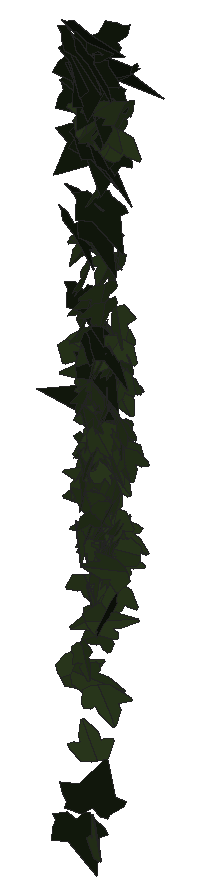
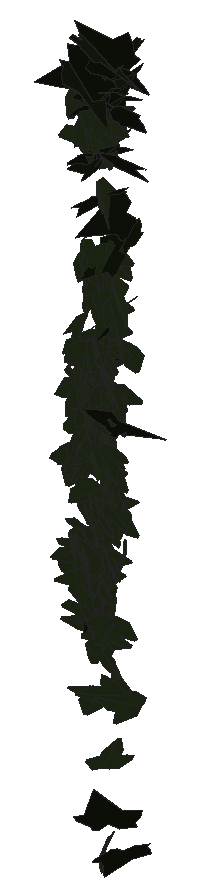
# SketchUp Ruby script. Lengths in inches.
U = 1.inch
M = Sketchup.active_model
def pt(a) = Geom::Point3d.new(a.map { |v| v * U })
def face(e, loops, mat)
  f = e.add_face(loops[0].map { |a| pt(a) })
  loops[1..].each { |l| e.add_face(l.map { |a| pt(a) }).erase! }
  f.material = f.back_material = mat if mat
  f
end
# faces: each face lists its corners as indices into pts; further lists are holes
def faces(e, pts, list, mat = nil) = list.each { |f| face(e, (f[0].is_a?(Array) ? f : [f]).map { |l| l.map { |i| pts[i] } }, mat) }
# xy, xz, yz: faces in a plane at the given z, y or x. An outline is a flat list of corners, or four numbers for a rectangle; further outlines are holes
def ring(l) = l.size == 4 ? [[l[0], l[1]], [l[2], l[1]], [l[2], l[3]], [l[0], l[3]]] : l.each_slice(2).to_a
def flat(e, list, mat, &to3) = list.each { |f| face(e, (f[0].is_a?(Array) ? f : [f]).map { |l| ring(l).map { |u, v| to3.(u, v) } }, mat) }
def xy(e, z, list, mat = nil) = flat(e, list, mat) { |x, y| [x, y, z] }
def xz(e, y, list, mat = nil) = flat(e, list, mat) { |x, z| [x, y, z] }
def yz(e, x, list, mat = nil) = flat(e, list, mat) { |y, z| [x, y, z] }
def lines(e, pts, list) = list.each { |a, b| e.add_line(pt(pts[a]), pt(pts[b])) }
# prism: a flat outline (further loops are holes) pulled along v
def prism(e, loops, v, mat = nil)
  f = face(e, loops, mat); d = Geom::Vector3d.new(v.map { |x| x * U })
  f.pushpull(f.normal.samedirection?(d) ? d.length : -d.length)
end
def box(e, o, s, mat = nil) = prism(e, [[o, [o[0] + s[0], o[1], o[2]], [o[0] + s[0], o[1] + s[1], o[2]], [o[0], o[1] + s[1], o[2]]]], [0, 0, s[2]], mat)
def at(x, y, z, deg = 0) = Geom::Transformation.translation(pt([x, y, z])) * Geom::Transformation.rotation(ORIGIN, Z_AXIS, deg.degrees)
def axes(o, x, y, z) = Geom::Transformation.new([*x, 0, *y, 0, *z, 0, *pt(o).to_a, 1])
def part(name) = M.definitions.add(name)
# library, detail: a bought-in or finely detailed component or shape, given as its bounding box
def library(name, o, s) = part(name).tap { |d| box(d.entities, o, s) }
def detail(e, o, s) = box(e.add_group.entities, o, s)
def put(e, d, t, mat = nil) = e.add_instance(d, t).tap { |i| i.material = mat if mat }
def group(e, t, mat = nil) = e.add_group.tap { |g| g.transformation = t; g.material = mat if mat }.entities
root = M.entities
M.materials.add("1026 AP 7946 SUNNY SIDE UP").color = [254, 231, 186]
M.materials.add("efeu1").color = [18, 25, 13]
M.materials.add("efeu2").color = [43, 57, 29]
c1 = part("ivyleaf_10")
p = [[0,0.5,-0.03],[-0.0625,2.02,-0.43],[-0.19,2.01,-0.46],[-0.54,1.05,-0.29],[-0.52,0.625,-0.18],[-0.83,0.76,-0.28],
  [-1.16,0.64,-0.33],[-1.15,0.33,-0.24],[-0.77,-0.39,0.02],[-0.3,-0.51,0.16],[0.04,-0.48,0.23],[-0.02,2.01,-0.4375],
  [-0.06,2.01,-0.43],[0.04,-0.49,0.23],[0.67,-0.49,0.14],[1.38,0.36,-0.2],[1.375,0.51,-0.24],[0.81,0.65,-0.19],
  [0.62,0.59,-0.15],[0.6,1.09,-0.28],[0.5,1.23,-0.31]]
faces(c1.entities,p,[[0,1,2,3,4,5,6,7,8,9,10],[11,12,0,13,14,15,16,17,18,19,20]],"efeu2")
c2 = part("ivyleaf_9")
p = [[1.54,2.16,1.25],[1.36,2.04,1.19],[-0.21,0.99,0.68],[-0.71,1.11,0.82],[-0.85,0.86,0.67],[-0.8,0.17,0.21],
  [-0.9,-0.01,0.1],[-0.67,-0.16,-0.02],[-0.08,-0.08,-0.05],[-0.03,-0.6,-0.4],[0.65,-0.88,-0.66],[0.83,-0.6,-0.49],
  [1.29,-0.42,-0.43],[1.8125,-0.07,-0.26],[1.21,0.44,0.15]]
faces(c2.entities,p,[[0,1,2,3,4,5,6,7,8,9,10,11,12,13,14]],"efeu1")
put(root,c1,axes([106.875,212.88,260.41],[-0.19029,-0.14773,0.11261],[-0.06597,-0.10624,-0.19489],[0.28215,-0.12447,0.03039]),"1026 AP 7946 SUNNY SIDE UP")
put(root,c2,axes([107.1,212.89,261.68],[-0.24512,0.04227,0.19567],[-0.3019,0.00418,-0.16348],[-0.04735,-0.24549,0.02942]),"1026 AP 7946 SUNNY SIDE UP")
put(root,c1,axes([106.83,212.86,260.92],[-0.31168,0.09367,0.01752],[-0.03684,-0.01117,-0.22498],[-0.14494,-0.19859,0.0195]),"1026 AP 7946 SUNNY SIDE UP")
put(root,c1,axes([106.73,212.96,258.57],[-0.26839,-0.09301,-0.07264],[0.13434,-0.01575,-0.19319],[0.12429,-0.1838,0.05196]),"1026 AP 7946 SUNNY SIDE UP")
put(root,c1,axes([106.63,212.64,257.13],[0.09438,0.04793,-0.22139],[0.24114,0.15113,0.07963],[0.24902,-0.16451,0.0068]),"1026 AP 7946 SUNNY SIDE UP")
put(root,c1,axes([106.8125,212.81,260.76],[0.22467,-0.16796,0.00881],[-0.00657,-0.01601,-0.22684],[0.26444,0.1423,-0.01312]),"1026 AP 7946 SUNNY SIDE UP")
put(root,c1,axes([106.83,212.74,263.82],[0.11401,-0.23435,0.00026],[0.0017,-0.00132,-0.25272],[0.3685,0.07251,0.00109]),"1026 AP 7946 SUNNY SIDE UP")
put(root,c2,axes([106.7,212.92,267.24],[-0.06033,-0.19698,0.16164],[0.02129,-0.16121,-0.20458],[0.39651,-0.02131,0.03558]),"1026 AP 7946 SUNNY SIDE UP")
put(root,c1,axes([106.82,212.73,260.82],[-0.08581,0.21184,0.03996],[-0.04434,0.0314,-0.22431],[-0.33538,-0.05835,0.01943]),"1026 AP 7946 SUNNY SIDE UP")
put(root,c1,axes([106.86,212.83,262.19],[-0.24604,-0.16556,0.00822],[0.00748,-0.01674,-0.23427],[0.26059,-0.15583,0.01449]),"1026 AP 7946 SUNNY SIDE UP")
put(root,c1,axes([106.86,212.9,260.92],[-0.00747,-0.22363,-0.00585],[-0.00483,0.00447,-0.23038],[0.35166,-0.00469,-0.00329]),"1026 AP 7946 SUNNY SIDE UP")
put(root,c1,axes([106.77,212.95,262.59],[-0.16197,0.17997,-0.09615],[0.04265,-0.09266,-0.21312],[-0.31666,-0.10453,0.02047]),"1026 AP 7946 SUNNY SIDE UP")
put(root,c2,axes([106.64,212.77,267.67],[0.15307,-0.24266,0.02043],[-0.00058,-0.02299,-0.26933],[0.38301,0.09694,-0.00857]),"1026 AP 7946 SUNNY SIDE UP")
put(root,c2,axes([106.95,212.89,266.02],[-0.3785,-0.06932,-0.00194],[0.02255,-0.04449,-0.25379],[0.10667,-0.23657,0.04675]),"1026 AP 7946 SUNNY SIDE UP")
put(root,c1,axes([106.82,212.9,258.9],[-0.21299,0.15516,-0.01584],[0.00136,-0.02078,-0.21188],[-0.2453,-0.13483,0.01258]),"1026 AP 7946 SUNNY SIDE UP")
put(root,c1,axes([106.76,212.7,259.54],[-0.0639,0.19851,-0.12817],[0.03544,-0.12353,-0.20945],[-0.36761,-0.04642,0.00209]),"1026 AP 7946 SUNNY SIDE UP")
put(root,c1,axes([106.83,212.96,259.66],[0.14342,-0.19112,0.02627],[0.01622,-0.02453,-0.2183],[0.30298,0.09178,-0.00075]),"1026 AP 7946 SUNNY SIDE UP")
put(root,c1,axes([106.87,212.97,259.56],[-0.16054,-0.18227,0.03579],[0.01037,-0.04436,-0.21367],[0.29189,-0.09868,0.02728]),"1026 AP 7946 SUNNY SIDE UP")
put(root,c1,axes([106.89,212.85,264.41],[-0.02994,-0.19682,0.14607],[-0.01596,-0.14258,-0.20452],[0.38213,-0.02137,0.0029]),"1026 AP 7946 SUNNY SIDE UP")
put(root,c1,axes([106.89,213,259.29],[-0.09176,-0.19462,0.03705],[-0.00634,-0.03747,-0.20942],[0.31146,-0.0581,0.00666]),"1026 AP 7946 SUNNY SIDE UP")
put(root,c1,axes([106.86,212.93,264.49],[-0.1538,-0.22251,-0.06366],[0.05442,0.05085,-0.24985],[0.35848,-0.10318,0.01061]),"1026 AP 7946 SUNNY SIDE UP")
put(root,c1,axes([106.82,212.9,258.44],[-0.09357,0.19403,-0.03018],[0.00656,-0.03051,-0.20919],[-0.30874,-0.05945,0.0047]),"1026 AP 7946 SUNNY SIDE UP")
put(root,c2,axes([106.66,212.73,264.58],[0.10039,-0.19777,0.14375],[0.06086,-0.13528,-0.21485],[0.37671,0.07456,-0.0036]),"1026 AP 7946 SUNNY SIDE UP")
put(root,c2,axes([106.79,212.83,266.9],[-0.05764,-0.12549,0.22384],[-0.03673,-0.21764,-0.1344],[0.3938,-0.03867,0.02023]),"1026 AP 7946 SUNNY SIDE UP")
put(root,c2,axes([106.7,212.9,264.57],[0.32306,-0.13253,-0.05726],[-0.07283,0.02935,-0.2517],[0.21344,0.21061,0.00078]),"1026 AP 7946 SUNNY SIDE UP")
put(root,c1,axes([106.9,212.66,263.17],[0.12332,-0.21752,-0.044],[0.0002,0.04404,-0.23746],[0.34819,0.07701,0.01572]),"1026 AP 7946 SUNNY SIDE UP")
put(root,c1,axes([106.88,212.91,260.07],[-0.29785,0.09958,-0.02522],[0.02592,-0.02239,-0.22025],[-0.15936,-0.18976,0.01132]),"1026 AP 7946 SUNNY SIDE UP")
put(root,c1,axes([107.06,212.62,262.05],[-0.27734,0.09266,0.12943],[-0.20342,0.01796,-0.20148],[-0.1362,-0.2155,0.03736]),"1026 AP 7946 SUNNY SIDE UP")
put(root,c1,axes([106.89,212.76,260.12],[-0.32683,-0.04574,-0.03259],[0.05394,-0.01036,-0.21859],[0.06855,-0.20995,0.0166]),"1026 AP 7946 SUNNY SIDE UP")
put(root,c2,axes([106.7,212.76,265.12],[0.36817,-0.07574,-0.00511],[-0.00424,0.00639,-0.25343],[0.11924,0.2341,0.00678]),"1026 AP 7946 SUNNY SIDE UP")
put(root,c2,axes([106.79,212.64,254.71],[-0.0297,-0.22602,-0.09822],[0.02553,0.09298,-0.23297],[0.38409,-0.02365,0.00789]),"1026 AP 7946 SUNNY SIDE UP")
put(root,c1,axes([106.89,212.97,259.24],[-0.07735,-0.19475,0.04909],[0.08021,-0.06068,-0.19702],[0.30533,-0.0334,0.0642]),"1026 AP 7946 SUNNY SIDE UP")
put(root,c1,axes([106.96,212.67,261.98],[0.03385,-0.23664,0.016],[-0.00236,-0.01708,-0.24488],[0.37304,0.02137,-0.003]),"1026 AP 7946 SUNNY SIDE UP")
put(root,c1,axes([106.93,212.8,262.29],[0.17732,-0.20113,0.02047],[0.00895,-0.02089,-0.23761],[0.31785,0.11279,-0.00473]),"1026 AP 7946 SUNNY SIDE UP")
put(root,c1,axes([106.95,212.56,260.36],[0.14897,-0.18169,-0.09819],[-0.01013,0.10119,-0.20697],[0.3217,0.08732,0.03895]),"1026 AP 7946 SUNNY SIDE UP")
put(root,c1,axes([106.92,212.92,262.8],[-0.04274,0.22618,0.01962],[-0.03349,0.01526,-0.23376],[-0.35517,-0.02866,0.01968]),"1026 AP 7946 SUNNY SIDE UP")
put(root,c1,axes([106.97,212.94,261.29],[0.33624,0.00031,-0.06747],[-0.10153,0.03846,-0.21677],[0.01725,0.22031,0.03926]),"1026 AP 7946 SUNNY SIDE UP")
put(root,c1,axes([106.98,212.65,263.45],[-0.02373,-0.23584,-0.00858],[0.00184,0.00693,-0.24341],[0.37099,-0.01512,0.00066]),"1026 AP 7946 SUNNY SIDE UP")
put(root,c1,axes([107.05,212.86,258.17],[0.0938,0.07416,-0.18861],[-0.19686,-0.1343,-0.09863],[-0.24103,0.13855,0.00716]),"1026 AP 7946 SUNNY SIDE UP")
put(root,c1,axes([106.97,212.71,260.84],[0.04979,-0.16342,-0.17953],[0.01601,0.17564,-0.16764],[0.37425,0.01423,0.03106]),"1026 AP 7946 SUNNY SIDE UP")
put(root,c1,axes([106.78,212.72,257.55],[0.19392,-0.06096,0.15494],[0.20835,-0.07198,-0.14209],[0.1482,0.18098,-0.00298]),"1026 AP 7946 SUNNY SIDE UP")
put(root,c1,axes([106.97,212.81,266.59],[-0.13246,-0.18428,0.15838],[0.04374,-0.17036,-0.19433],[0.37588,-0.04511,0.07843]),"1026 AP 7946 SUNNY SIDE UP")
put(root,c1,axes([106.92,213,259.3],[-0.08049,0.14506,-0.14378],[0.01611,-0.14278,-0.15667],[-0.31701,-0.04409,0.02855]),"1026 AP 7946 SUNNY SIDE UP")
put(root,c1,axes([107.08,212.98,259.58],[-0.30723,0.00362,0.07405],[-0.11153,-0.04462,-0.19662],[0.019,-0.20335,0.04321]),"1026 AP 7946 SUNNY SIDE UP")
put(root,c2,axes([107.24,212.93,267.75],[-0.28959,0.17928,0.02162],[-0.0941,-0.0338,-0.25617],[-0.26758,-0.18214,0.06669]),"1026 AP 7946 SUNNY SIDE UP")
put(root,c1,axes([106.91,213.01,259.29],[0.20346,-0.14102,0.08381],[0.08078,-0.06432,-0.19747],[0.24358,0.13912,-0.00452]),"1026 AP 7946 SUNNY SIDE UP")
put(root,c1,axes([107.17,212.75,257.9375],[-0.20498,0.0587,0.15321],[-0.24335,0.00021,-0.14015],[-0.06117,-0.19752,0.04412]),"1026 AP 7946 SUNNY SIDE UP")
put(root,c1,axes([106.99,212.89,262.75],[0.162,-0.205,0.01846],[-0.00097,-0.02164,-0.23625],[0.32374,0.10252,-0.00994]),"1026 AP 7946 SUNNY SIDE UP")
put(root,c2,axes([106.83,212.74,263.5],[0.07723,-0.23826,-0.01681],[0.00159,0.01549,-0.25049],[0.37537,0.04895,0.00452]),"1026 AP 7946 SUNNY SIDE UP")
put(root,c2,axes([106.71,212.93,267.61],[0.03453,-0.11597,0.23289],[0.26498,-0.16399,-0.10419],[0.30021,0.15809,0.06517]),"1026 AP 7946 SUNNY SIDE UP")
put(root,c1,axes([107.01,212.9375,259.71],[0.11923,-0.2002,-0.02236],[-0.00484,0.02082,-0.22037],[0.31641,0.07576,0.00505]),"1026 AP 7946 SUNNY SIDE UP")
put(root,c2,axes([106.88,212.81,266.79],[-0.23049,-0.12029,-0.17045],[0.22534,0.08369,-0.19379],[0.22831,-0.20404,0.01919]),"1026 AP 7946 SUNNY SIDE UP")
put(root,c1,axes([107.02,212.5625,261.65],[-0.28885,0.13019,0.00558],[-0.02396,-0.01345,-0.23114],[-0.20344,-0.18327,0.0193]),"1026 AP 7946 SUNNY SIDE UP")
put(root,c1,axes([106.97,213.02,259.32],[-0.10353,0.19599,-0.02435],[0.00237,-0.02559,-0.21303],[-0.31061,-0.06552,0.00649]),"1026 AP 7946 SUNNY SIDE UP")
put(root,c1,axes([107.22,212.73,262.71],[0.03844,-0.00163,-0.25329],[-0.24968,0.18853,-0.01645],[0.29516,0.15969,0.01907]),"1026 AP 7946 SUNNY SIDE UP")
put(root,c1,axes([107.24,212.9,260.26],[0.10419,-0.06817,-0.23777],[-0.27386,0.15104,-0.09675],[0.2603,0.18619,-0.00662]),"1026 AP 7946 SUNNY SIDE UP")
put(root,c1,axes([107.05,212.88,262.89],[0.06171,-0.23228,-0.00252],[0.0013,0.00128,-0.24268],[0.36524,0.03924,0.00129]),"1026 AP 7946 SUNNY SIDE UP")
put(root,c1,axes([106.84,212.53,262.75],[-0.16671,-0.10976,-0.18567],[0.29094,0.04728,-0.14201],[0.15779,-0.20314,0.06567]),"1026 AP 7946 SUNNY SIDE UP")
put(root,c2,axes([106.87,212.72,266.16],[0.19454,-0.21273,-0.07781],[-0.05362,0.06614,-0.25311],[0.35025,0.12828,0.00447]),"1026 AP 7946 SUNNY SIDE UP")
put(root,c1,axes([107.06,212.9,261.09],[0.06259,-0.21767,0.03943],[0.01034,-0.03896,-0.22818],[0.3477,0.04034,-0.00031]),"1026 AP 7946 SUNNY SIDE UP")
put(root,c1,axes([107.09,212.88,261.91],[-0.17518,-0.18259,0.08696],[0.00076,-0.09787,-0.21537],[0.31698,-0.10067,0.04858]),"1026 AP 7946 SUNNY SIDE UP")
put(root,c2,axes([107.07,212.9,266.96],[-0.29119,-0.17519,0.01232],[0.0312,-0.03955,-0.25921],[0.27445,-0.18138,0.04253]),"1026 AP 7946 SUNNY SIDE UP")
put(root,c2,axes([106.98,212.69,267.38],[-0.30916,-0.08232,-0.16531],[0.24271,0.04461,-0.2188],[0.14539,-0.24953,0.01375]),"1026 AP 7946 SUNNY SIDE UP")
put(root,c1,axes([107.1,212.79,266.3],[-0.01825,-0.25506,0.02821],[-0.00073,-0.02884,-0.2632],[0.40361,-0.01158,0.0008]),"1026 AP 7946 SUNNY SIDE UP")
put(root,c1,axes([107.08,212.77,265.34],[0.0921,-0.24595,-0.02436],[-0.00258,0.02248,-0.2603],[0.3883,0.05848,0.00405]),"1026 AP 7946 SUNNY SIDE UP")
put(root,c1,axes([107.11,212.59,263.06],[-0.0779,-0.23396,-0.03149],[0.00821,0.02878,-0.2462],[0.37066,-0.04981,-0.00116]),"1026 AP 7946 SUNNY SIDE UP")
put(root,c1,axes([107.07,212.7,262.81],[-0.17999,0.20583,-0.00602],[-0.01103,-0.01192,-0.24239],[-0.32365,-0.11406,0.01161]),"1026 AP 7946 SUNNY SIDE UP")
put(root,c1,axes([107.18,212.84,262.82],[0.13309,-0.16861,-0.1382],[-0.11654,0.11145,-0.19322],[0.31712,0.11172,-0.01301]),"1026 AP 7946 SUNNY SIDE UP")
put(root,c1,axes([107.12,212.6,256.01],[0.15553,0.208,0.0165],[-0.02774,-0.00801,0.23688],[0.32671,-0.0997,0.01226]),"1026 AP 7946 SUNNY SIDE UP")
put(root,c2,axes([107.07,212.64,255.08],[-0.27132,-0.05023,0.17508],[0.25865,0.04391,0.18538],[-0.10482,0.23838,0.00425]),"1026 AP 7946 SUNNY SIDE UP")
put(root,c1,axes([107.16,212.73,262.78],[-0.2758,-0.14165,0.03983],[-0.02967,-0.03925,-0.23171],[0.2293,-0.17545,0.01793]),"1026 AP 7946 SUNNY SIDE UP")
put(root,c1,axes([107.14,212.98,258.99],[-0.06114,-0.20357,0.01763],[0.00268,-0.01892,-0.21355],[0.32137,-0.03857,0.00514]),"1026 AP 7946 SUNNY SIDE UP")
put(root,c1,axes([107.08,212.86,259.31],[0.20451,-0.15025,0.05997],[0.03929,-0.0562,-0.20428],[0.25079,0.13132,-0.01689]),"1026 AP 7946 SUNNY SIDE UP")
put(root,c1,axes([107.15,212.93,261.85],[-0.13403,-0.21096,-0.0025],[0.01138,-0.0016,-0.23429],[0.33152,-0.08524,0.00703]),"1026 AP 7946 SUNNY SIDE UP")
put(root,c2,axes([106.9,212.77,267.48],[0.10752,-0.21467,0.13759],[0.07275,-0.12668,-0.23279],[0.39186,0.08242,0.00546]),"1026 AP 7946 SUNNY SIDE UP")
put(root,c1,axes([107.12,212.78,258.91],[0.0614,0.18786,-0.08039],[-0.048,-0.07425,-0.1976],[-0.3169,0.04764,0.01435]),"1026 AP 7946 SUNNY SIDE UP")
put(root,c1,axes([106.89,212.64,257.18],[0.05133,0.02548,0.22125],[0.2849,0.1151,-0.0418],[-0.18526,0.18407,-0.00297]),"1026 AP 7946 SUNNY SIDE UP")
put(root,c1,axes([107.11,212.69,261.49],[0.08141,-0.18179,0.13574],[0.0745,-0.12441,-0.19521],[0.34606,0.06955,0.01009]),"1026 AP 7946 SUNNY SIDE UP")
put(root,c1,axes([107.19,213.01,259.56],[-0.07523,-0.20378,0.0043],[-0.00052,-0.0054,-0.21567],[0.32053,-0.04783,0.00066]),"1026 AP 7946 SUNNY SIDE UP")
put(root,c1,axes([107.22,212.8,266.6875],[-0.07824,-0.22061,0.11325],[-0.03212,-0.10935,-0.23359],[0.38713,-0.05366,0.00351]),"1026 AP 7946 SUNNY SIDE UP")
put(root,c1,axes([107.2,212.76,262.13],[-0.11758,-0.21683,0.03231],[-0.00682,-0.03297,-0.23639],[0.34471,-0.07462,0.00635]),"1026 AP 7946 SUNNY SIDE UP")
put(root,c1,axes([107.19,212.6875,266.42],[0.37106,-0.03707,-0.08098],[-0.10906,0.05575,-0.24191],[0.08186,0.24234,0.04479]),"1026 AP 7946 SUNNY SIDE UP")
put(root,c1,axes([107.1875,212.98,262.85],[-0.25351,-0.16099,0.02945],[0.02995,-0.05958,-0.22808],[0.2556,-0.15269,0.05593]),"1026 AP 7946 SUNNY SIDE UP")
put(root,c1,axes([107.18,213.01,259.55],[0.07349,-0.20198,-0.03268],[-0.0014,0.03117,-0.2133],[0.32121,0.04634,0.00655]),"1026 AP 7946 SUNNY SIDE UP")
put(root,c2,axes([107.34,212.86,267.18],[-0.05532,0.25314,0.0332],[-0.07577,0.02392,-0.2592],[-0.39375,-0.04017,0.04521]),"1026 AP 7946 SUNNY SIDE UP")
put(root,c1,axes([107.18,212.9,260.43],[0.21458,-0.16901,-0.02442],[-0.02544,0.01617,-0.22368],[0.26693,0.1374,-0.00169]),"1026 AP 7946 SUNNY SIDE UP")
put(root,c2,axes([107.1,212.89,266.01],[-0.13414,-0.23643,-0.00553],[0.01675,0.00043,-0.25874],[0.37144,-0.08541,0.00967]),"1026 AP 7946 SUNNY SIDE UP")
put(root,c1,axes([107.15,212.7,262.6875],[0.14328,-0.19688,0.09873],[0.0589,-0.08948,-0.22399],[0.34001,0.09847,-0.0028]),"1026 AP 7946 SUNNY SIDE UP")
put(root,c2,axes([107.09,212.93,266.84],[-0.08432,-0.2459,0.02286],[0.00011,-0.02415,-0.25936],[0.38843,-0.05337,0.00504]),"1026 AP 7946 SUNNY SIDE UP")
put(root,c1,axes([107.22,213.01,259.59],[-0.02747,-0.20842,0.01169],[-0.00606,-0.01225,-0.21552],[0.32825,-0.01767,-0.003]),"1026 AP 7946 SUNNY SIDE UP")
put(root,c2,axes([107.12,212.59,262.97],[0.13523,-0.14255,-0.18512],[-0.15561,0.14911,-0.17056],[0.32426,0.13101,-0.00465]),"1026 AP 7946 SUNNY SIDE UP")
put(root,c1,axes([106.96,212.75,261.02],[-0.09203,-0.06623,-0.2144],[0.31776,0.0643,-0.0794],[0.12876,-0.20603,0.0427]),"1026 AP 7946 SUNNY SIDE UP")
put(root,c1,axes([107.22,213,259.28],[-0.02563,-0.20565,0.0269],[0.00041,-0.02738,-0.21267],[0.3262,-0.01612,0.00238]),"1026 AP 7946 SUNNY SIDE UP")
put(root,c1,axes([107.21,212.88,261.83],[0.03809,-0.2255,0.0098],[0.00767,-0.01033,-0.23368],[0.3549,0.02443,0.004]),"1026 AP 7946 SUNNY SIDE UP")
put(root,c1,axes([107.2,212.8,259.02],[0.22232,-0.16087,-0.01417],[-0.02177,0.00492,-0.22049],[0.25282,0.14189,-0.00652]),"1026 AP 7946 SUNNY SIDE UP")
put(root,c1,axes([107.27,212.49,254.45],[-0.08543,0.1937,-0.1355],[-0.0465,0.1294,0.20794],[0.3662,0.06162,-0.00521]),"1026 AP 7946 SUNNY SIDE UP")
put(root,c2,axes([107.0625,212.71,262.51],[0.05585,-0.22889,-0.08197],[-0.00993,0.0782,-0.2381],[0.38024,0.03566,0.00582]),"1026 AP 7946 SUNNY SIDE UP")
put(root,c1,axes([107.23,212.84,260.05],[0.13016,-0.20435,0.00486],[-0.00752,-0.00827,-0.22705],[0.32137,0.08257,-0.00728]),"1026 AP 7946 SUNNY SIDE UP")
put(root,c1,axes([107.16,212.55,262.8],[-0.12917,-0.17984,-0.1477],[0.14105,0.11396,-0.201],[0.33192,-0.11842,0.02794]),"1026 AP 7946 SUNNY SIDE UP")
put(root,c1,axes([107.28,212.85,262.07],[-0.20871,-0.1812,0.0343],[-0.01494,-0.03551,-0.23121],[0.28961,-0.13242,0.01279]),"1026 AP 7946 SUNNY SIDE UP")
put(root,c1,axes([107.1875,212.5,260.07],[-0.11439,-0.15666,-0.15218],[0.10712,0.13018,-0.1771],[0.32017,-0.09953,0.00488]),"1026 AP 7946 SUNNY SIDE UP")
put(root,c1,axes([107.3,212.9375,262.18],[-0.35423,-0.02409,0.03508],[-0.04876,-0.02951,-0.23207],[0.04414,-0.22594,0.0252]),"1026 AP 7946 SUNNY SIDE UP")
put(root,c1,axes([107.27,212.6,262.63],[0.1028,-0.22374,-0.05806],[-0.01542,0.05451,-0.23974],[0.36199,0.06586,0.00628]),"1026 AP 7946 SUNNY SIDE UP")
put(root,c1,axes([107.29,212.83,264.2],[-0.0978,-0.21205,0.09785],[-0.00278,-0.09913,-0.22688],[0.36611,-0.05739,0.02441]),"1026 AP 7946 SUNNY SIDE UP")
put(root,c1,axes([107.29,212.61,263.8],[-0.10182,-0.22992,-0.01563],[0.00735,0.01309,-0.246],[0.36211,-0.06491,0.0006]),"1026 AP 7946 SUNNY SIDE UP")
put(root,c2,axes([107.1,212.65,264.79],[0.08713,-0.23705,-0.01763],[-0.00003,0.01619,-0.25067],[0.37356,0.05529,0.00409]),"1026 AP 7946 SUNNY SIDE UP")
put(root,c1,axes([107.05,212.94,260.625],[0.2289,0.09188,0.14302],[0.19724,0.05967,-0.1765],[-0.17107,0.19173,-0.01212]),"1026 AP 7946 SUNNY SIDE UP")
put(root,c1,axes([107.28,212.89,266.38],[-0.06047,-0.2493,0.00616],[0.02703,-0.01011,-0.25922],[0.39124,-0.03783,0.01886]),"1026 AP 7946 SUNNY SIDE UP")
put(root,c1,axes([107.49,212.99,259.29],[-0.00746,0.03085,0.21272],[-0.28659,-0.10098,0.01065],[0.15954,-0.17996,0.02908]),"1026 AP 7946 SUNNY SIDE UP")
put(root,c1,axes([107.31,212.59,263.52],[-0.09815,-0.22993,-0.01984],[0.0102,0.01684,-0.24534],[0.3625,-0.06273,0.00153]),"1026 AP 7946 SUNNY SIDE UP")
put(root,c1,axes([107.23,212.5625,261.39],[0.06965,0.2026,0.09348],[-0.01668,0.0932,-0.21118],[-0.34792,0.03609,0.02884]),"1026 AP 7946 SUNNY SIDE UP")
put(root,c1,axes([107.43,212.8125,261.48],[-0.21307,0.13563,0.12354],[-0.20559,0.029,-0.18702],[-0.19574,-0.17809,0.06196]),"1026 AP 7946 SUNNY SIDE UP")
put(root,c1,axes([107.33,212.87,261.5],[-0.32432,0.08555,0.02621],[-0.04454,-0.00329,-0.22961],[-0.13285,-0.20773,0.013]),"1026 AP 7946 SUNNY SIDE UP")
put(root,c1,axes([107.31,212.875,262.53],[0.09771,-0.21477,-0.0741],[-0.00181,0.07302,-0.22913],[0.35553,0.0594,0.0192]),"1026 AP 7946 SUNNY SIDE UP")
put(root,c1,axes([107.31,212.84,266.22],[0.38207,0.03259,-0.06362],[-0.09747,-0.00368,-0.25254],[-0.05109,0.25072,0.00606]),"1026 AP 7946 SUNNY SIDE UP")
put(root,c2,axes([107.08,212.81,265.91],[0.20505,-0.21771,0.02302],[0.00589,-0.02522,-0.2614],[0.34428,0.1301,-0.00924]),"1026 AP 7946 SUNNY SIDE UP")
put(root,c1,axes([107.27,212.95,258.6],[0.32488,-0.00667,-0.01952],[-0.03048,-0.01605,-0.21237],[0.00812,0.20685,-0.01589]),"1026 AP 7946 SUNNY SIDE UP")
put(root,c1,axes([107.375,212.92,262.64],[-0.25913,0.14539,0.07086],[-0.11111,0.02172,-0.22427],[-0.22657,-0.17693,0.02894]),"1026 AP 7946 SUNNY SIDE UP")
put(root,c1,axes([107.33,212.9,262.48],[-0.00387,-0.22559,-0.04368],[0.01512,0.04099,-0.23199],[0.36025,-0.00415,0.00927]),"1026 AP 7946 SUNNY SIDE UP")
put(root,c1,axes([107.26,212.97,259.12],[0.23499,0.14417,0.01405],[-0.00011,0.01851,-0.21337],[-0.22759,0.14885,0.01462]),"1026 AP 7946 SUNNY SIDE UP")
put(root,c2,axes([107.16,212.66,265.19],[0.02014,-0.23537,-0.08176],[0.03964,0.07896,-0.24066],[0.38788,0.00415,0.02884]),"1026 AP 7946 SUNNY SIDE UP")
put(root,c2,axes([107.03,212.89,267.33],[0.36379,-0.01404,0.11195],[0.16914,-0.02019,-0.23856],[0.03345,0.25485,-0.01123]),"1026 AP 7946 SUNNY SIDE UP")
put(root,c1,axes([107.26,212.9,259.875],[0.32678,-0.04037,0.02926],[0.03662,-0.02928,-0.21685],[0.06866,0.20773,-0.02359]),"1026 AP 7946 SUNNY SIDE UP")
put(root,c1,axes([107.4,212.76,260.32],[0.15826,-0.18223,-0.11184],[-0.06286,0.10055,-0.21351],[0.32671,0.10762,0.01309]),"1026 AP 7946 SUNNY SIDE UP")
put(root,c1,axes([107.32,212.96,259.71],[0.06366,-0.19343,0.08198],[0.05036,-0.0755,-0.20347],[0.32568,0.04948,0.01543]),"1026 AP 7946 SUNNY SIDE UP")
put(root,c1,axes([107.3,212.86,260.92],[-0.06201,0.21801,0.0026],[0.00122,0.00145,-0.22822],[-0.3428,-0.03943,-0.00128]),"1026 AP 7946 SUNNY SIDE UP")
put(root,c1,axes([107.16,212.63,258.18],[-0.08085,-0.03273,0.21835],[0.20852,0.16669,0.06058],[-0.26541,0.14093,-0.01892]),"1026 AP 7946 SUNNY SIDE UP")
put(root,c1,axes([107.39,212.53,261.93],[0.0478,-0.15526,-0.16807],[-0.02353,0.16198,-0.16161],[0.35234,0.03188,0.01201]),"1026 AP 7946 SUNNY SIDE UP")
put(root,c1,axes([107.42,212.8125,261.16],[0.04203,0.0405,-0.24784],[-0.04638,0.241,0.03979],[0.38114,0.02486,0.03217]),"1026 AP 7946 SUNNY SIDE UP")
put(root,c1,axes([107.57,212.57,259.21],[0.13819,-0.01261,-0.21133],[-0.30931,0.05919,-0.09026],[0.09321,0.21511,0.01381]),"1026 AP 7946 SUNNY SIDE UP")
put(root,c1,axes([107.38,213.01,259.73],[0.06715,-0.20509,0.01711],[-0.00649,-0.019,-0.21577],[0.32363,0.04217,-0.00788]),"1026 AP 7946 SUNNY SIDE UP")
put(root,c1,axes([107.29,212.89,262.08],[-0.29711,-0.1125,-0.07568],[0.15074,-0.02551,-0.2158],[0.14724,-0.20089,0.06822]),"1026 AP 7946 SUNNY SIDE UP")
put(root,c2,axes([107.23,212.63,262.95],[0.17475,-0.21545,-0.06962],[-0.06594,0.05294,-0.2491],[0.3483,0.11812,-0.01223]),"1026 AP 7946 SUNNY SIDE UP")
put(root,c1,axes([107.43,212.75,262.83],[0.19766,0.1377,-0.1364],[-0.14069,-0.09865,-0.19266],[-0.26635,0.1543,0.00054]),"1026 AP 7946 SUNNY SIDE UP")
put(root,c1,axes([107.42,212.71,264.25],[0.03555,-0.2316,-0.08867],[0.01388,0.08582,-0.23865],[0.38753,0.01817,0.01668]),"1026 AP 7946 SUNNY SIDE UP")
put(root,c1,axes([107.45,212.88,261.09],[-0.23564,-0.15738,0.051],[-0.00737,-0.06396,-0.22049],[0.25974,-0.14459,0.04001]),"1026 AP 7946 SUNNY SIDE UP")
put(root,c1,axes([107.22,213.01,259.6],[-0.20991,-0.03978,-0.16183],[0.25393,-0.01974,-0.13655],[0.01628,-0.20503,0.04329]),"1026 AP 7946 SUNNY SIDE UP")
put(root,c1,axes([107.375,212.87,263.25],[-0.01101,0.23098,-0.02097],[-0.02017,-0.02203,-0.23779],[-0.36423,-0.00576,0.0138]),"1026 AP 7946 SUNNY SIDE UP")
put(root,c1,axes([107.38,212.88,262.25],[0.33112,-0.09669,0.00964],[0.00508,-0.01667,-0.23839],[0.15275,0.21015,-0.01297]),"1026 AP 7946 SUNNY SIDE UP")
put(root,c2,axes([107.52,212.4,258.56],[-0.06398,0.02512,-0.25697],[-0.27299,0.17968,0.04884],[0.2847,0.17794,-0.01092]),"1026 AP 7946 SUNNY SIDE UP")
put(root,c1,axes([107.46,212.81,266.78],[-0.08912,-0.24379,0.06812],[0.00009,-0.06919,-0.25778],[0.39776,-0.0546,0.01532]),"1026 AP 7946 SUNNY SIDE UP")
put(root,c1,axes([107.28,212.57,257.05],[0.26722,0.11612,0.07829],[0.11194,0.02899,-0.21129],[-0.18666,0.18362,-0.01462]),"1026 AP 7946 SUNNY SIDE UP")
put(root,c1,axes([107.39,212.95,261.3],[0.00983,-0.19885,-0.10464],[0.08949,0.09858,-0.19681],[0.33867,-0.02028,0.05504]),"1026 AP 7946 SUNNY SIDE UP")
put(root,c1,axes([107.42,212.89,260.98],[-0.34236,-0.03136,-0.03358],[0.05486,-0.01581,-0.22573],[0.04494,-0.21956,0.01973]),"1026 AP 7946 SUNNY SIDE UP")
